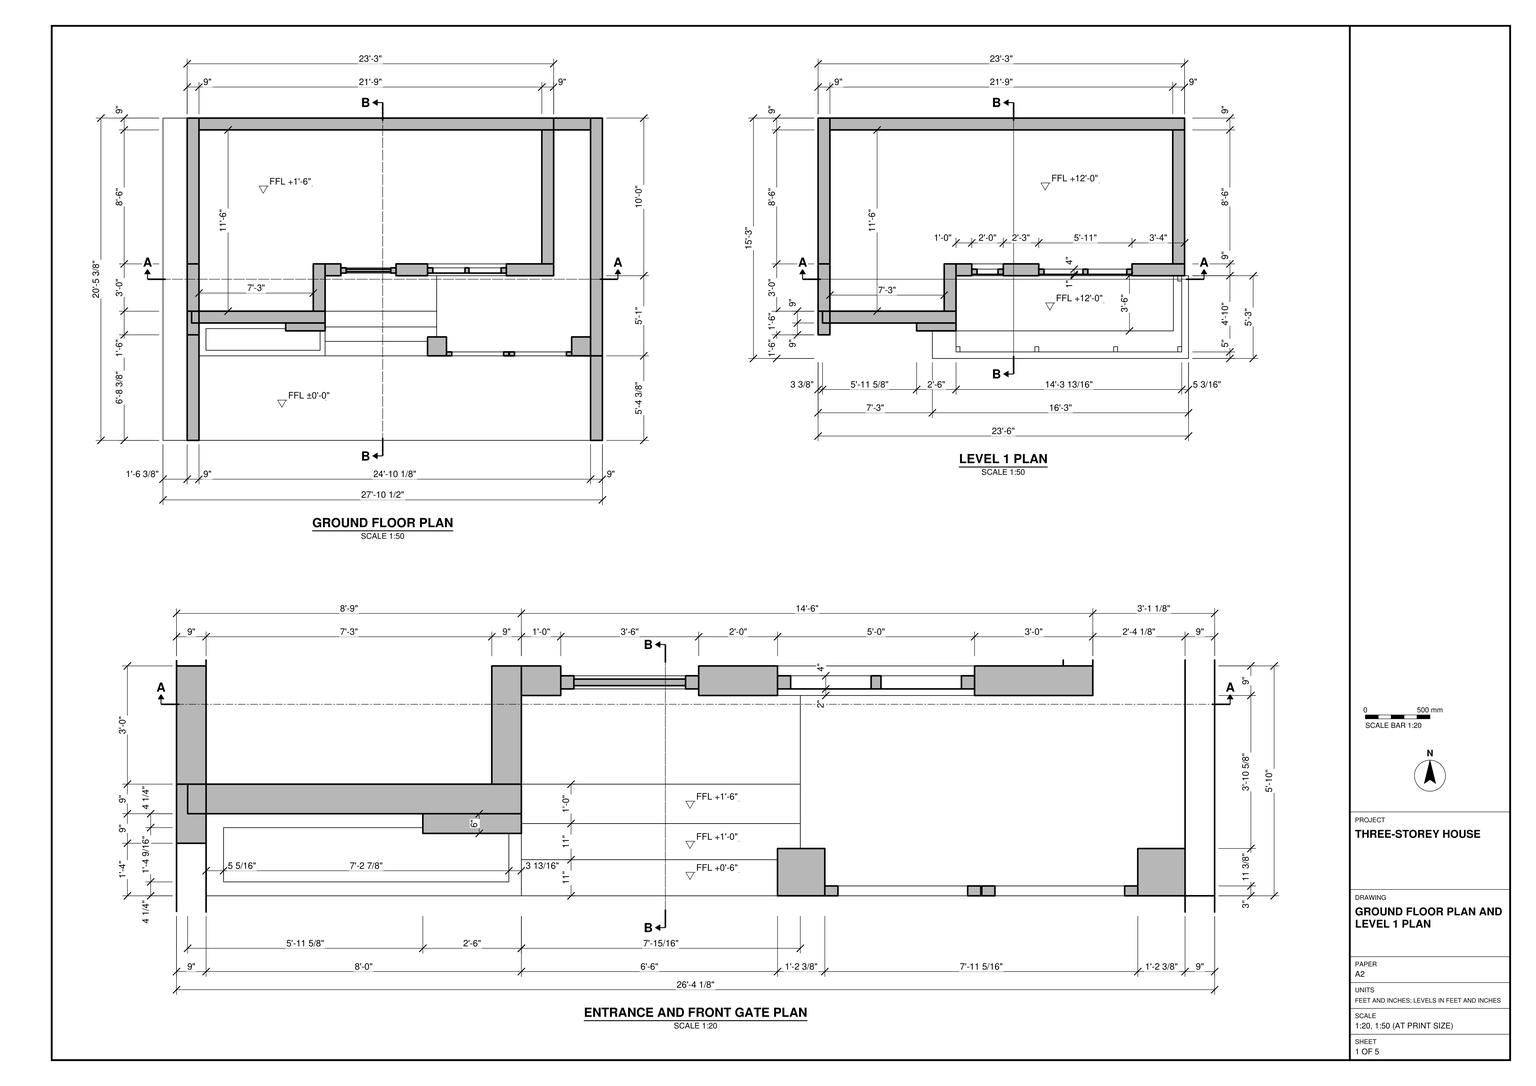
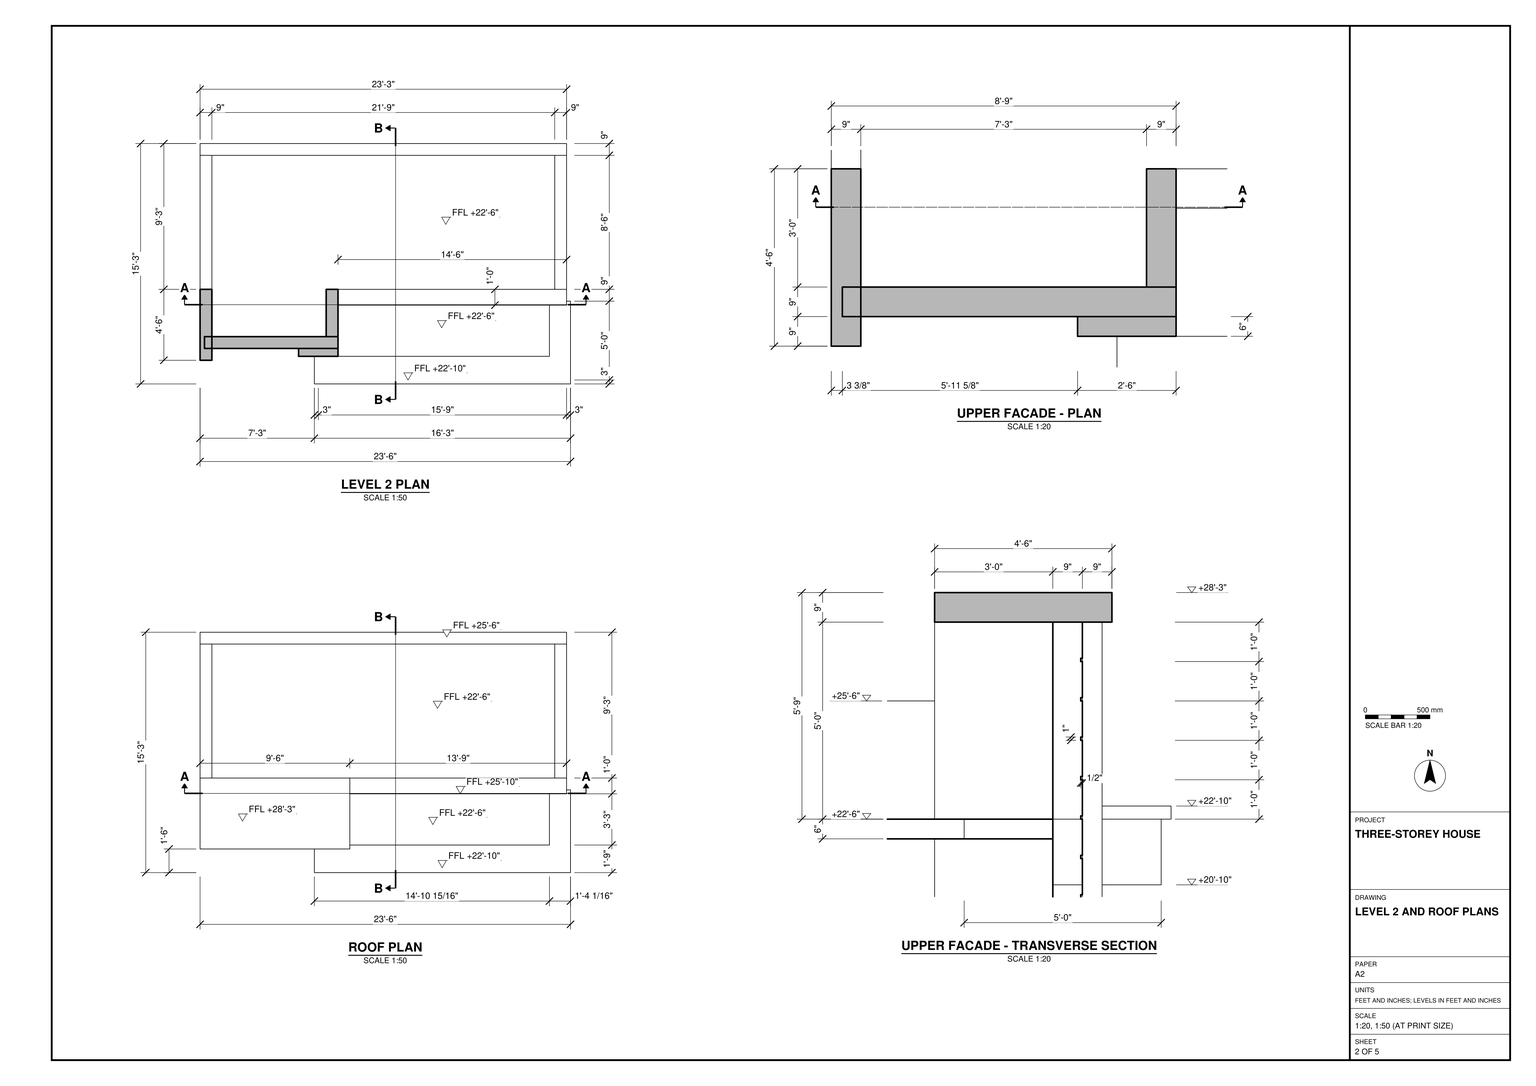
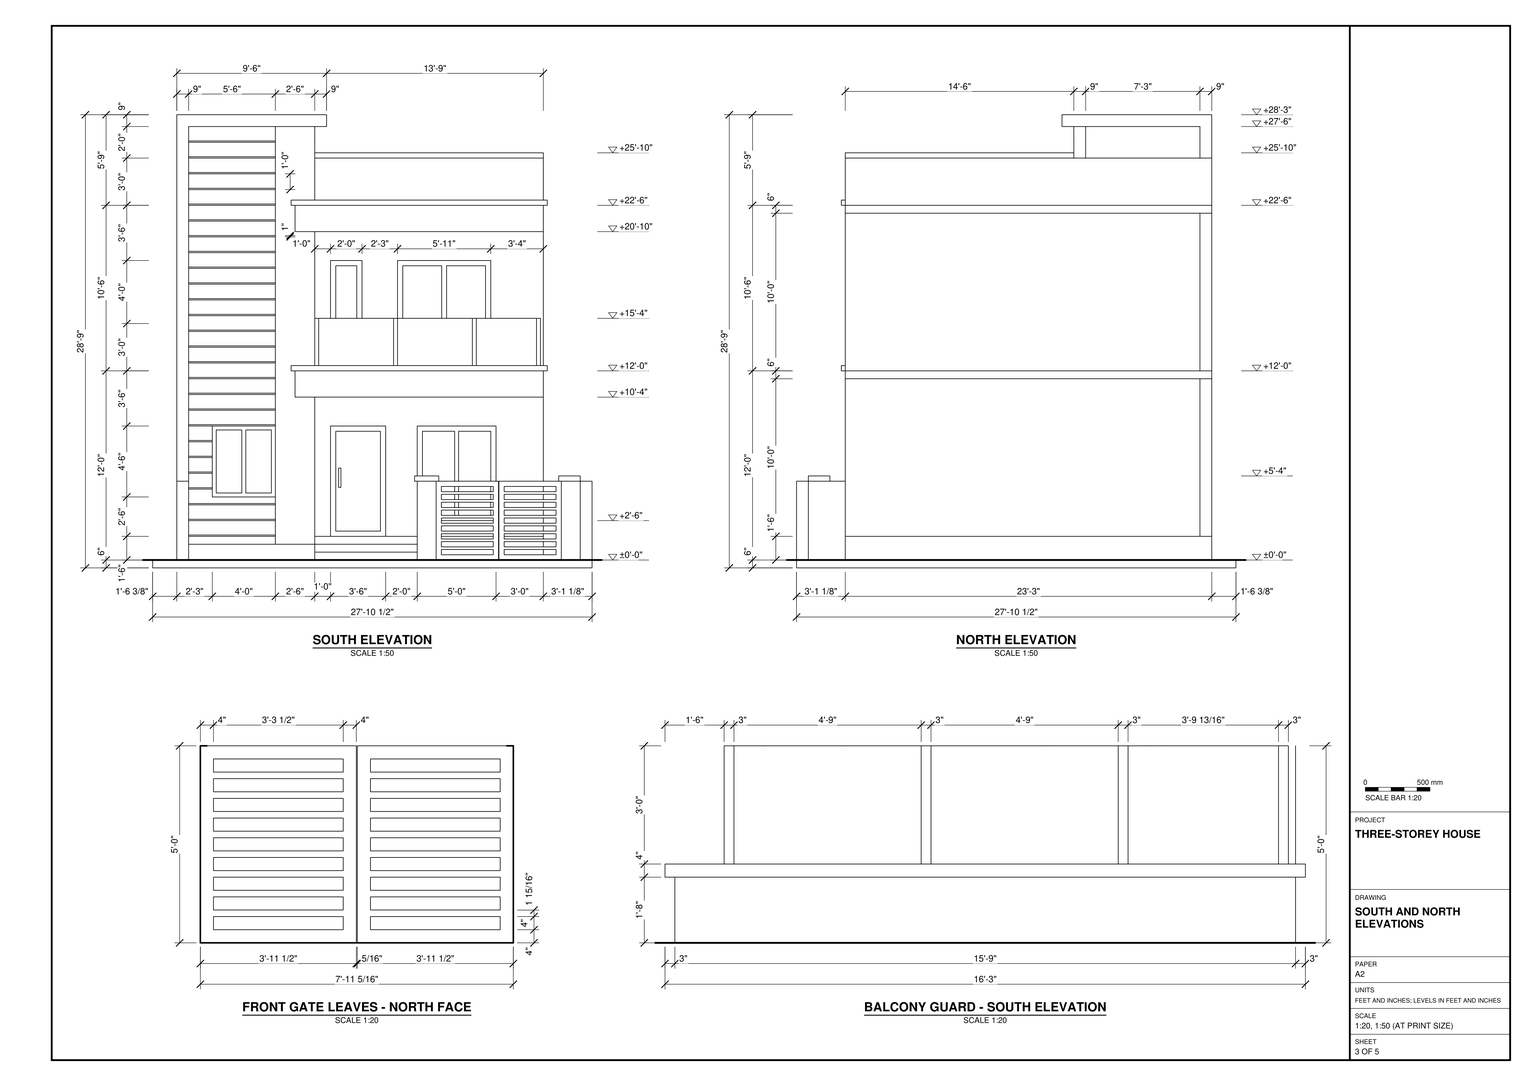
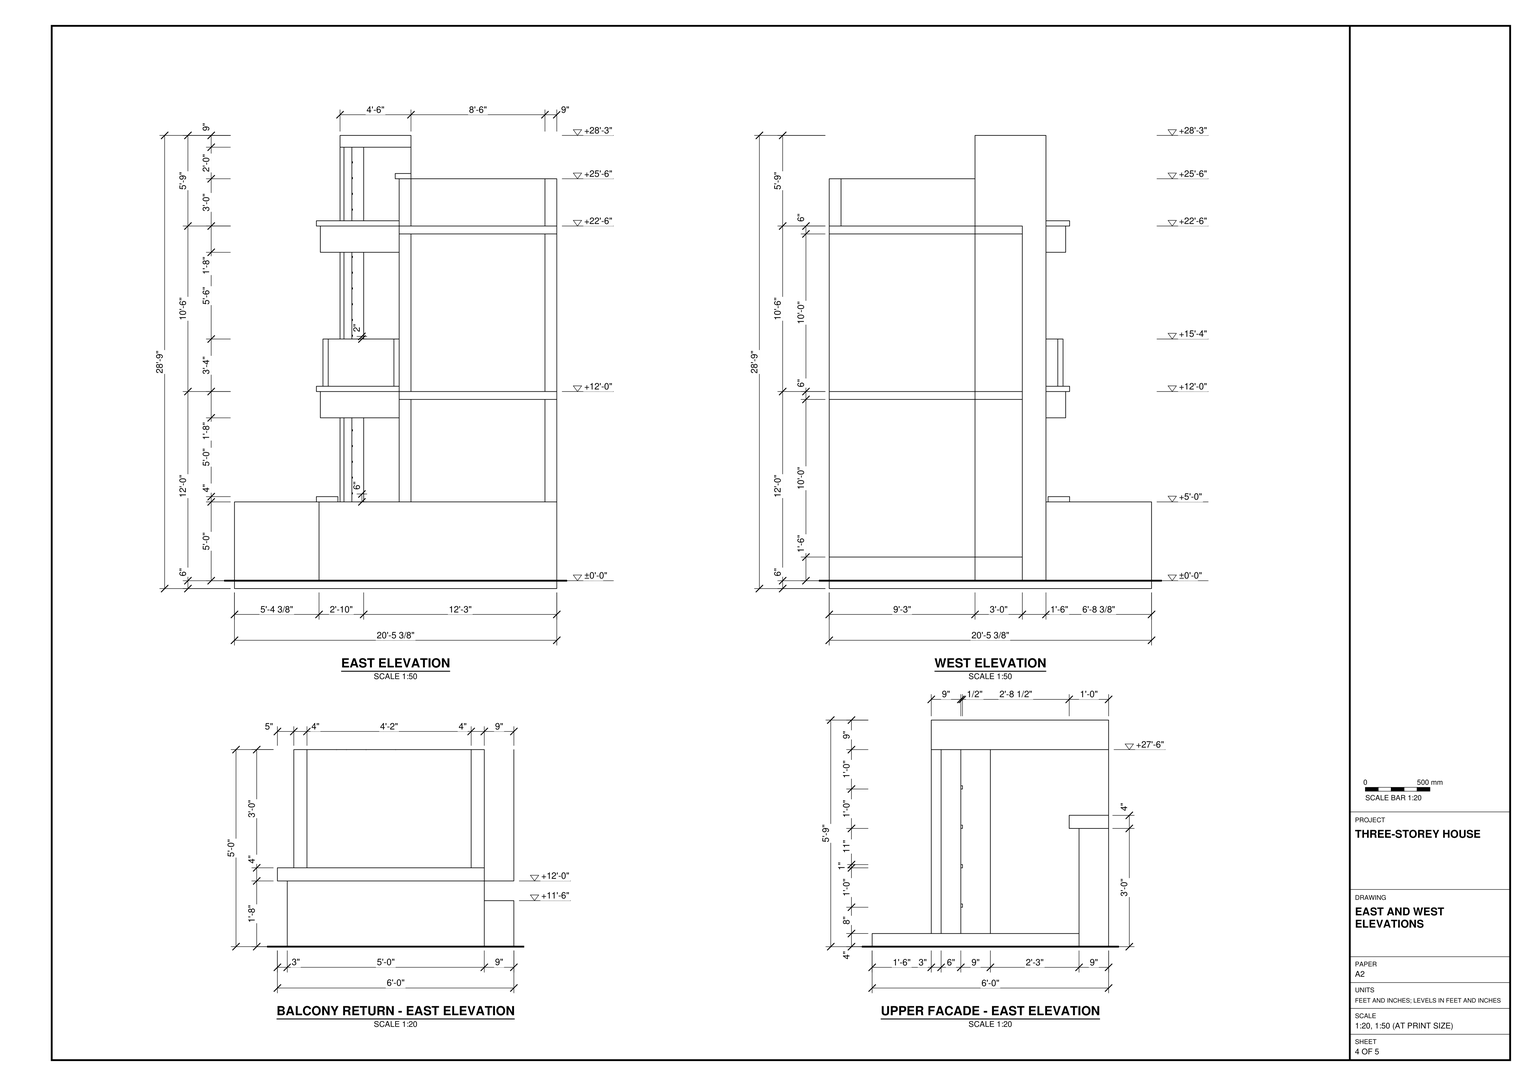
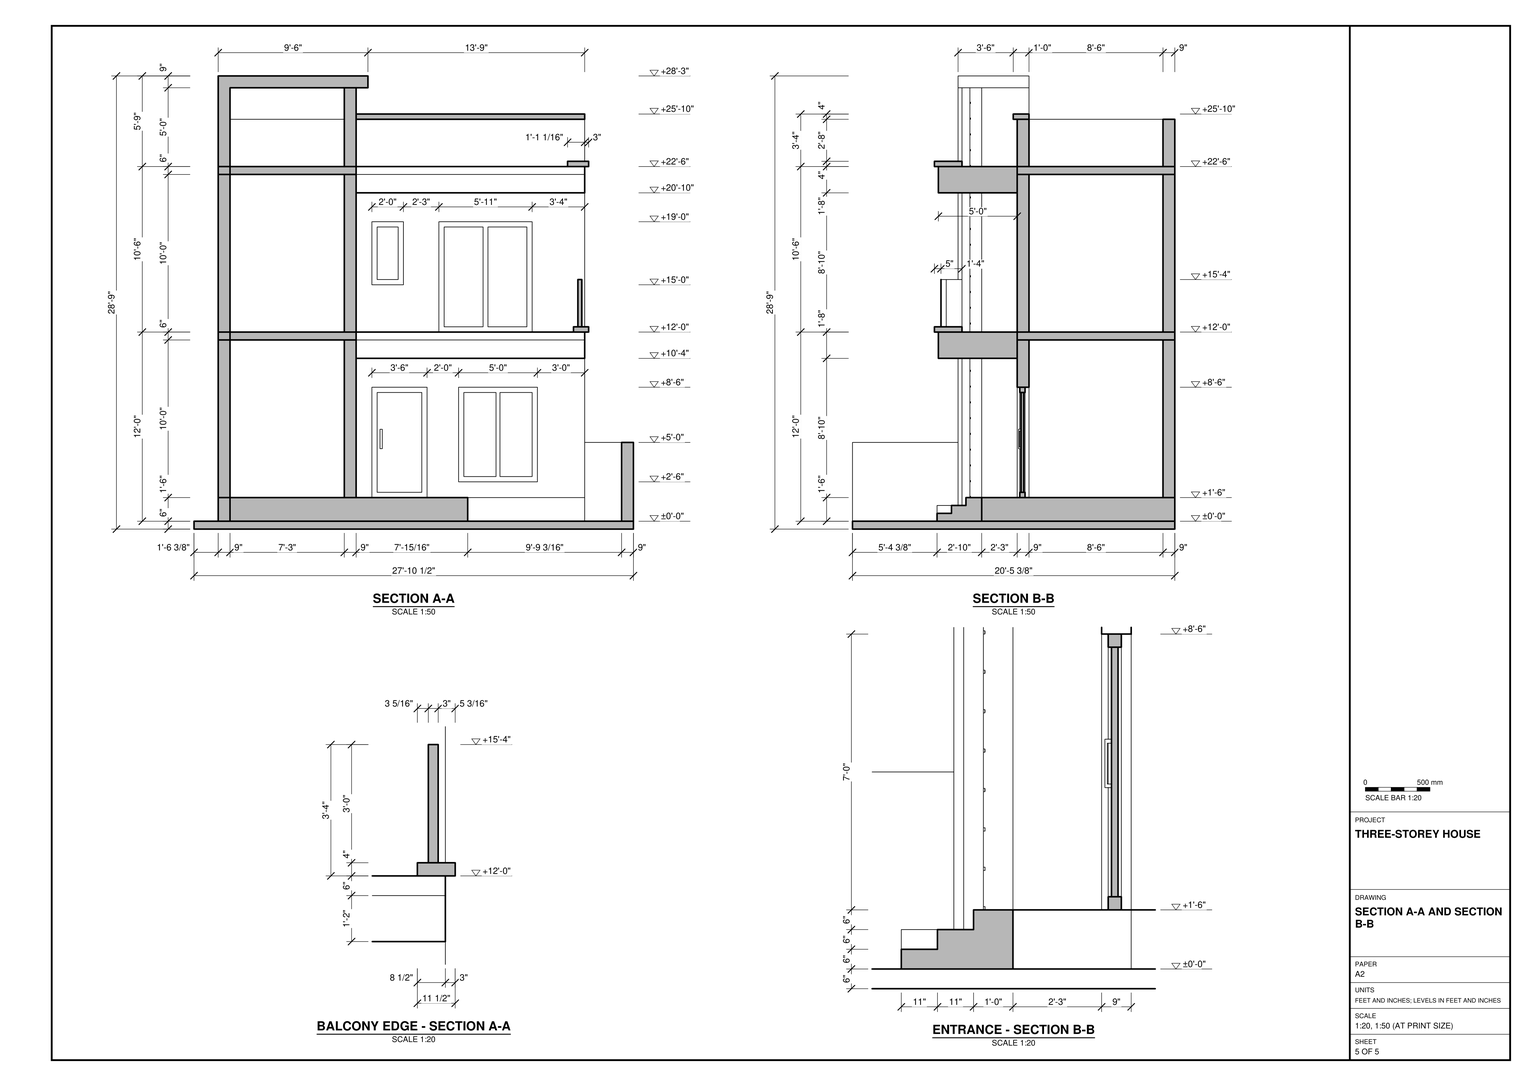
Build the house shown in task_files/diagram_01.pdf in SketchUp. Work in feet and inches. The complete model, including the base and entrance enclosure, measures 27'-10 1/2" across the south elevation, 20'-5 3/8" from front to back and 28'-9" high. Use ±0'-0" as the ground datum, with Level 1 at +12'-0" and Level 2 at +22'-6".

Follow the stepped footprint in plan, using 9" walls where indicated. Model the base, floor slabs and raised ground floor. Run the entrance steps up to the door landing at +1'-6", with the two-leaf gate between posts to the right of the steps. On the south face, distinguish the tall, horizontally banded bay on the left from the recessed door and window wall beneath the balcony. Model the openings and their frames, the projecting balcony slab and its panelled guard. Use the roof plan and transverse section to shape the flat roof, parapets and projecting cap over the tall bay.

Keep shell elements such as walls, slabs and roof separate as groups or components. Treat each furniture or joinery piece shown as a separate group or component, and use components for repeated parts. Decor and loose items may be any suitable library components. Save one SketchUp model as output_files/three_storey_house_with_a_balcony_and_gated_entrance.skp.

# SketchUp Ruby script. Lengths in inches.
U = 1.inch
M = Sketchup.active_model
def pt(a) = Geom::Point3d.new(a.map { |v| v * U })
def face(e, loops, mat)
  f = e.add_face(loops[0].map { |a| pt(a) })
  loops[1..].each { |l| e.add_face(l.map { |a| pt(a) }).erase! }
  f.material = f.back_material = mat if mat
  f
end
# faces: each face lists its corners as indices into pts; further lists are holes
def faces(e, pts, list, mat = nil) = list.each { |f| face(e, (f[0].is_a?(Array) ? f : [f]).map { |l| l.map { |i| pts[i] } }, mat) }
# xy, xz, yz: faces in a plane at the given z, y or x. An outline is a flat list of corners, or four numbers for a rectangle; further outlines are holes
def ring(l) = l.size == 4 ? [[l[0], l[1]], [l[2], l[1]], [l[2], l[3]], [l[0], l[3]]] : l.each_slice(2).to_a
def flat(e, list, mat, &to3) = list.each { |f| face(e, (f[0].is_a?(Array) ? f : [f]).map { |l| ring(l).map { |u, v| to3.(u, v) } }, mat) }
def xy(e, z, list, mat = nil) = flat(e, list, mat) { |x, y| [x, y, z] }
def xz(e, y, list, mat = nil) = flat(e, list, mat) { |x, z| [x, y, z] }
def yz(e, x, list, mat = nil) = flat(e, list, mat) { |y, z| [x, y, z] }
def lines(e, pts, list) = list.each { |a, b| e.add_line(pt(pts[a]), pt(pts[b])) }
# prism: a flat outline (further loops are holes) pulled along v
def prism(e, loops, v, mat = nil)
  f = face(e, loops, mat); d = Geom::Vector3d.new(v.map { |x| x * U })
  f.pushpull(f.normal.samedirection?(d) ? d.length : -d.length)
end
def box(e, o, s, mat = nil) = prism(e, [[o, [o[0] + s[0], o[1], o[2]], [o[0] + s[0], o[1] + s[1], o[2]], [o[0], o[1] + s[1], o[2]]]], [0, 0, s[2]], mat)
def at(x, y, z, deg = 0) = Geom::Transformation.translation(pt([x, y, z])) * Geom::Transformation.rotation(ORIGIN, Z_AXIS, deg.degrees)
def axes(o, x, y, z) = Geom::Transformation.new([*x, 0, *y, 0, *z, 0, *pt(o).to_a, 1])
def part(name) = M.definitions.add(name)
# library, detail: a bought-in or finely detailed component or shape, given as its bounding box
def library(name, o, s) = part(name).tap { |d| box(d.entities, o, s) }
def detail(e, o, s) = box(e.add_group.entities, o, s)
def put(e, d, t, mat = nil) = e.add_instance(d, t).tap { |i| i.material = mat if mat }
def group(e, t, mat = nil) = e.add_group.tap { |g| g.transformation = t; g.material = mat if mat }.entities
root = M.entities
M.materials.add("[Color M07]").color = [58, 58, 58]
M.materials.add("[Grass Dark Green]").color = [106, 157, 55]
M.materials.add("[Stone Brushed Khaki]").color = [229, 239, 196]
M.materials.add("[Translucent Glass Blue]").color = [51, 76, 122]
M.materials["[Translucent Glass Blue]"].alpha = 0.5
M.materials.add("[Translucent Glass Gray]").color = [71, 71, 71]
M.materials["[Translucent Glass Gray]"].alpha = 0.5
M.materials.add("[Translucent Glass Gray]1").color = [0, 0, 0]
M.materials["[Translucent Glass Gray]1"].alpha = 0.5
M.materials.add("[Wood Cherry Original]").color = [112, 63, 31]
M.materials.add("[Wood Veneer 01]").color = [76, 44, 23]
c1 = part("Group\#40")
box(c1.entities,[0,0,0],[3,4,36])
g1 = group(root,at(0,139,0))
box(g1,[0,-139,0],[334.5,245.37,6])
g2 = group(root,at(57.4,5.37,6))
prism(g2,[[[240,240,0],[240,120,0],[150.9375,120,0],[150.9375,93,0],[66,93,0],[-39,93,0],[-39,240,0]]],[0,0,18])
g3 = group(root,at(57.4,125.37,24))
prism(g3,[[[78,9,0],[66,9,0],[66,9,120],[240,9,120],[240,9,0],[120,9,0],[120,9,84],[78,9,84]],[[204,9,12],[204,9,84],[144,9,84],[144,9,12]]],[0,-9,0])
g4 = group(root,at(201.4,127.37,36),"[Wood Veneer 01]")
prism(g4,[[[0,0,72],[0,0,0],[60,0,0],[60,0,72]],[[28.5,0,68],[28.5,0,4],[4,0,4],[4,0,68]],[[31.5,0,68],[56,0,68],[56,0,4],[31.5,0,4]]],[0,4,0])
g5 = group(root,at(232.9,127.37,40),"[Translucent Glass Gray]")
xz(g5,0,[[0,0,24.5,64]])
g6 = group(root,at(205.4,127.37,40),"[Translucent Glass Gray]1")
xz(g6,0,[[0,0,24.5,64]])
g7 = group(root,at(135.4,127.37,24),"[Wood Veneer 01]")
prism(g7,[[[42,4,0],[0,4,0],[0,4,84],[42,4,84]],[[38,4,4],[38,4,80],[4,4,80],[4,4,4]]],[0,-4,0])
g8 = group(root,at(139.4,128.37,28),"[Wood Veneer 01]")
box(g8,[0,0,0],[34,2,76])
g9 = group(root,at(46.27,89.37,6),"[Wood Veneer 01]")
xy(g9,0,[[-24.5,0,77.125,9]])
xy(g9,6,[[-24.5,0,77.125,0.5]])
xy(g9,7,[[-24.5,0,77.125,0.5]])
xy(g9,18,[[-24.5,0,77.125,0.5]])
xy(g9,19,[[-24.5,0,77.125,0.5]])
xy(g9,30,[[-24.5,0,77.125,0.5]])
xy(g9,31,[[-24.5,0,77.125,0.5]])
xy(g9,42,[[-24.5,0,77.125,0.5]])
xy(g9,43,[[-24.5,0,77.125,0.5]])
xy(g9,48,[[-0.875,0,47.125,9]])
xy(g9,54,[[-24.5,0,-0.875,0.5],[47.125,0,77.125,0.4375]])
xy(g9,55,[[-24.5,0,-0.875,0.5],[47.125,0,77.125,0.4375]])
xy(g9,66,[[-24.5,0,-0.875,0.5],[47.125,0,77.125,0.4375]])
xy(g9,67,[[-24.5,0,-0.875,0.5],[47.125,0,77.125,0.4375]])
xy(g9,78,[[-24.5,0,-0.875,0.5],[47.125,0,77.125,0.4375]])
xy(g9,79,[[-24.5,0,-0.875,0.5],[47.125,0,77.125,0.4375]])
xy(g9,90,[[-24.5,0,-0.875,0.5],[47.125,0,77.125,0.4375]])
xy(g9,91,[[-24.5,0,-0.875,0.5],[47.125,0,77.125,0.4375]])
xy(g9,102,[[-24.5,0,-1.16,0.5],[-1.16,0,-0.875,0.5],[47.33,0,77.125,0.4375],[-0.875,0.5,47.125,9]])
xy(g9,103,[[-24.5,0,-1.16,0.5],[-1.16,0,47.125,0.5],[47.33,0,77.125,0.4375]])
xy(g9,114,[[-24.5,0,77.125,0.5]])
xy(g9,115,[[-24.5,0,77.125,0.5]])
xy(g9,126,[[-24.5,0,77.125,0.5]])
xy(g9,127,[[-24.5,0,77.125,0.5]])
xy(g9,138,[[-24.5,0,77.125,0.5]])
xy(g9,139,[[-24.5,0,77.125,0.5]])
xy(g9,150,[[-24.5,0,77.125,0.5]])
xy(g9,151,[[-24.5,0,77.125,0.5]])
xy(g9,162,[[-24.5,0,77.125,0.5]])
xy(g9,163,[[-24.5,0,77.125,0.5]])
xy(g9,174,[[-24.5,0,77.125,0.5]])
xy(g9,175,[[-24.5,0,77.125,0.5]])
xy(g9,186,[[-24.5,0,77.125,0.5]])
xy(g9,187,[[-24.5,0,77.125,0.5]])
xy(g9,198,[[-24.5,0,77.125,0.5]])
xy(g9,199,[[-24.5,0,77.125,0.5]])
xy(g9,210,[[-24.5,0,77.125,0.5]])
xy(g9,211,[[-24.5,0,77.125,0.5]])
xy(g9,222,[[-24.5,0,77.125,0.5]])
xy(g9,223,[[-24.5,0,77.125,0.5]])
xy(g9,234,[[-24.5,0,77.125,0.5]])
xy(g9,235,[[-24.5,0,77.125,0.5]])
xy(g9,246,[[-24.5,0,77.125,0.5]])
xy(g9,247,[[-24.5,0,77.125,0.5]])
xy(g9,258,[[-24.5,0,77.125,0.5]])
xy(g9,259,[[-24.5,0,77.125,0.5]])
xy(g9,270,[[-24.5,0,77.125,0.5]])
xy(g9,271,[[-24.5,0,77.125,0.5]])
xy(g9,282,[[-24.5,0,77.125,0.5]])
xy(g9,283,[[-24.5,0,77.125,0.5]])
xy(g9,294,[[-24.5,0,77.125,0.5]])
xy(g9,295,[[-24.5,0,77.125,0.5]])
xy(g9,306,[[-24.5,0,77.125,0.5]])
xy(g9,307,[[-24.5,0,77.125,0.5]])
xy(g9,318,[[-24.5,0,77.125,0.5]])
xy(g9,319,[[-24.5,0,77.125,0.5]])
xy(g9,330,[[-24.5,0,77.125,9]])
xz(g9,0,[[-24.5,0,77.125,6],[-24.5,7,77.125,18],[-24.5,19,77.125,30],[-24.5,31,77.125,42],[-24.5,43,77.125,43,77.125,54,47.125,54,47.125,48,-0.875,48,-0.875,54,-24.5,54],
  [-24.5,55,-0.875,66],[47.125,55,77.125,66],[-24.5,67,-0.875,78],[47.125,67,77.125,78],[-24.5,79,-0.875,90],
  [47.125,79,77.125,90],[-24.5,91,-0.875,102],[47.125,91,77.125,91,77.125,102,47.33,102,47.33,103,77.125,103,77.125,114,-24.5,114,-24.5,103,47.125,103],[-24.5,115,77.125,126],[-24.5,127,77.125,138],
  [-24.5,139,77.125,150],[-24.5,151,77.125,162],[-24.5,163,77.125,174],[-24.5,175,77.125,186],[-24.5,187,77.125,198],
  [-24.5,199,77.125,210],[-24.5,211,77.125,222],[-24.5,223,77.125,234],[-24.5,235,77.125,246],[-24.5,247,77.125,258],
  [-24.5,259,77.125,270],[-24.5,271,77.125,282],[-24.5,283,77.125,294],[-24.5,295,77.125,306],[-24.5,307,77.125,318],
  [-24.5,319,77.125,330]])
xz(g9,0.4375,[[47.125,54,77.125,55],[47.125,66,77.125,67],[47.125,78,77.125,79],[47.125,90,77.125,91],[47.33,102,77.125,103]])
xz(g9,0.5,[[-24.5,6,77.125,7],[-24.5,18,77.125,19],[-24.5,30,77.125,31],[-24.5,42,77.125,43],[-24.5,54,-0.875,55],
  [-24.5,66,-0.875,67],[-24.5,78,-0.875,79],[-24.5,90,-0.875,91],[-24.5,102,47.125,103],[-24.5,114,77.125,115],
  [-24.5,126,77.125,127],[-24.5,138,77.125,139],[-24.5,150,77.125,151],[-24.5,162,77.125,163],[-24.5,174,77.125,175],
  [-24.5,186,77.125,187],[-24.5,198,77.125,199],[-24.5,210,77.125,211],[-24.5,222,77.125,223],[-24.5,234,77.125,235],
  [-24.5,246,77.125,247],[-24.5,258,77.125,259],[-24.5,270,77.125,271],[-24.5,282,77.125,283],[-24.5,294,77.125,295],
  [-24.5,306,77.125,307],[-24.5,318,77.125,319]])
xz(g9,9,[[[-24.5,0,77.125,330],[-0.875,48,47.125,102]]])
yz(g9,-24.5,[[0,0,0,6,0.5,6,0.5,7,0,7,0,18,0.5,18,0.5,19,0,19,0,30,0.5,30,0.5,31,0,31,0,42,0.5,42,0.5,43,0,43,0,54,0.5,54,0.5,55,0,55,0,66,0.5,66,0.5,67,0,67,0,78,0.5,78,0.5,79,0,79,0,90,0.5,90,0.5,91,0,91,0,102,0.5,102,0.5,103,0,103,0,114,0.5,114,0.5,115,0,115,0,126,0.5,126,0.5,127,0,127,0,138,0.5,138,0.5,139,0,139,0,150,0.5,150,0.5,151,0,151,0,162,0.5,162,0.5,163,0,163,0,174,0.5,174,0.5,175,0,175,0,186,0.5,186,0.5,187,0,187,0,198,0.5,198,0.5,199,0,199,0,210,0.5,210,0.5,211,0,211,0,222,0.5,222,0.5,223,0,223,0,234,0.5,234,0.5,235,0,235,0,246,0.5,246,0.5,247,0,247,0,258,0.5,258,0.5,259,0,259,0,270,0.5,270,0.5,271,0,271,0,282,0.5,282,0.5,283,0,283,0,294,0.5,294,0.5,295,0,295,0,306,0.5,306,0.5,307,0,307,0,318,0.5,318,0.5,319,0,319,0,330,9,330,9,0]])
yz(g9,-0.875,[[0,48,9,48,9,102,0,102,0,91,0.5,91,0.5,90,0,90,0,79,0.5,79,0.5,78,0,78,0,67,0.5,67,0.5,66,0,66,0,55,0.5,55,0.5,54,0,54]])
yz(g9,47.125,[[0,48,0,54,0.4375,54,0.4375,55,0,55,0,66,0.4375,66,0.4375,67,0,67,0,78,0.4375,78,0.4375,79,0,79,0,90,0.4375,90,0.4375,91,0,91,0,102,9,102,9,48],[0,102,0.5,103]])
yz(g9,47.33,[[0,102,0.4375,103]])
yz(g9,77.125,[[0,0,9,0,9,330,0,330,0,319,0.5,319,0.5,318,0,318,0,307,0.5,307,0.5,306,0,306,0,295,0.5,295,0.5,294,0,294,0,283,0.5,283,0.5,282,0,282,0,271,0.5,271,0.5,270,0,270,0,259,0.5,259,0.5,258,0,258,0,247,0.5,247,0.5,246,0,246,0,235,0.5,235,0.5,234,0,234,0,223,0.5,223,0.5,222,0,222,0,211,0.5,211,0.5,210,0,210,0,199,0.5,199,0.5,198,0,198,0,187,0.5,187,0.5,186,0,186,0,175,0.5,175,0.5,174,0,174,0,163,0.5,163,0.5,162,0,162,0,151,0.5,151,0.5,150,0,150,0,139,0.5,139,0.5,138,0,138,0,127,0.5,127,0.5,126,0,126,0,115,0.5,115,0.5,114,0,114,0,103,0.4375,103,0.4375,102,0,102,0,91,0.4375,91,0.4375,90,0,90,0,79,0.4375,79,0.4375,78,0,78,0,67,0.4375,67,0.4375,66,0,66,0,55,0.4375,55,0.4375,54,0,54,0,43,0.5,43,0.5,42,0,42,0,31,0.5,31,0.5,30,0,30,0,19,0.5,19,0.5,18,0,18,0,7,0.5,7,0.5,6,0,6]])
g10 = group(root,at(114.4,98.37,24),"[Wood Veneer 01]")
box(g10,[0,0,0],[9,36,120])
g11 = group(root,at(45.4,93.87,54),"[Wood Cherry Original]")
prism(g11,[[[48,4,54],[48,4,0],[0,4,0],[0,4,54]],[[22.5,4,3],[22.5,4,51],[3,4,51],[3,4,3]],[[45,4,51],[25.5,4,51],[25.5,4,3],[45,4,3]]],[0,-4,0])
g12 = group(root,at(70.9,93.87,57),"[Translucent Glass Gray]1")
xz(g12,0,[[0,0,19.5,48]])
g13 = group(root,at(48.4,93.87,57),"[Translucent Glass Gray]1")
xz(g13,0,[[0,0,19.5,48]])
g14 = group(root,at(18.4,98.37,24))
box(g14,[0,0,0],[9,147,120])
g15 = group(root,at(27.4,236.37,24))
box(g15,[0,0,0],[270,9,120])
g16 = group(root,at(288.4,134.37,24))
box(g16,[0,0,0],[9,102,120])
g17 = group(root,at(18.4,98.37,144))
prism(g17,[[[279,147,0],[279,27,0],[105,27,0],[105,0,0],[0,0,0],[0,147,0]]],[0,0,6])
g18 = group(root,at(123.4,89.37,130))
xy(g18,0,[[-15,-24,-15,-6,0,-6,0,36,174,36,174,-24]],"[Wood Veneer 01]")
xy(g18,20,[[-15,-24,174,-24,174,36,0,36,0,-6,-15,-6]])
xz(g18,-24,[[-15,0,174,20]])
xz(g18,-6,[[-15,0,0,20]])
xz(g18,36,[[0,0,174,20]])
yz(g18,-15,[[-24,0,-6,20]])
yz(g18,0,[[-6,0,36,20]])
yz(g18,174,[[-24,0,36,20]])
g19 = group(root,at(123.4,125.37,150))
prism(g19,[[[63,9,0],[0,9,0],[0,9,120],[174,9,120],[174,9,0],[134,9,0],[134,9,84],[63,9,84]],[[36,9,36],[36,9,84],[12,9,84],[12,9,36]]],[0,-9,0])
g20 = group(root,at(186.4,126.37,150),"[Wood Veneer 01]")
prism(g20,[[[71,4,0],[0,4,0],[0,4,84],[71,4,84]],[[33.65,4,4],[33.65,4,80],[4,4,80],[4,4,4]],[[67,4,80],[37.35,4,80],[37.35,4,4],[67,4,4]]],[0,-4,0])
g21 = group(root,at(223.75,126.37,154),"[Translucent Glass Blue]")
xz(g21,0,[[0,0,29.65,76]])
g22 = group(root,at(190.4,126.37,154),"[Translucent Glass Blue]")
xz(g22,0,[[0,0,29.65,76]])
g23 = group(root,at(135.4,126.37,186),"[Wood Veneer 01]")
prism(g23,[[[0,0,48],[0,0,0],[24,0,0],[24,0,48]],[[20,0,44],[20,0,4],[4,0,4],[4,0,44]]],[0,4,0])
g24 = group(root,at(139.4,126.37,190),"[Translucent Glass Blue]")
xz(g24,0,[[0,0,16,40]])
g25 = group(root,at(114.4,98.37,150),"[Wood Veneer 01]")
box(g25,[0,0,0],[9,36,120])
g26 = group(root,at(18.4,98.37,150))
box(g26,[0,0,0],[9,147,120])
g27 = group(root,at(27.4,236.37,150))
box(g27,[0,0,0],[270,9,120])
g28 = group(root,at(288.4,134.37,150))
box(g28,[0,0,0],[9,102,120])
g29 = group(root,at(18.4,98.37,270))
prism(g29,[[[0,147,0],[279,147,0],[279,27,0],[105,27,0],[105,0,0],[0,0,0]]],[0,0,6])
g30 = group(root,at(123.4,89.37,256))
xy(g30,0,[[-15,-24,-15,-6,0,-6,0,36,174,36,174,-24]],"[Wood Veneer 01]")
xy(g30,20,[[-15,-24,174,-24,174,36,0,36,0,-6,-15,-6]])
xz(g30,-24,[[-15,0,174,20]])
xz(g30,-6,[[-15,0,0,20]])
xz(g30,36,[[0,0,174,20]])
yz(g30,-15,[[-24,0,-6,20]])
yz(g30,0,[[-6,0,36,20]])
yz(g30,174,[[-24,0,36,20]])
g31 = group(root,at(123.4,125.37,276))
box(g31,[0,0,0],[174,9,36])
g32 = group(root,at(288.4,134.37,276))
box(g32,[0,0,0],[9,102,36])
g33 = group(root,at(18.4,236.37,276))
box(g33,[0,0,0],[279,9,36])
g34 = group(root,at(114.4,98.37,276),"[Wood Veneer 01]")
box(g34,[0,0,0],[9,36,60])
g35 = group(root,at(93.4,83.37,6),"[Wood Veneer 01]")
box(g35,[0,0,0],[30,6,330])
g36 = group(root,at(18.4,80.37,6))
prism(g36,[[[9,0,0],[9,0,330],[114,0,330],[114,0,339],[0,0,339],[0,0,0]]],[0,54,0])
g37 = group(root,at(108.4,65.37,276))
prism(g37,[[[-3,-3,0],[-3,18,0],[175.96,18,0],[175.96,60,0],[192,60,0],[192,-3,0]]],[0,0,4])
g38 = group(root,at(123.4,122.37,312))
box(g38,[0,0,0],[174,12,4])
g39 = group(root,at(108.4,65.37,150))
prism(g39,[[[192,60,0],[192,-3,0],[-3,-3,0],[-3,18,0],[180.47,18,0],[180.47,60,0]]],[0,0,4])
put(root,c1,at(123.4,67.37,154),"[Color M07]")
put(root,c1,at(183.4,67.37,154),"[Color M07]")
put(root,c1,at(243.4,67.37,154),"[Color M07]")
put(root,c1,at(292.21,67.37,154),"[Color M07]")
put(root,c1,at(292.21,121.37,154),"[Color M07]")
g40 = group(root,at(123.4,71.37,154),"[Translucent Glass Gray]1")
yz(g40,0,[[0,0,12,36]])
g41 = group(root,at(295.21,71.37,154),"[Translucent Glass Gray]1")
yz(g41,0,[[0,0,50,36]])
g42 = group(root,at(246.4,67.37,154),"[Translucent Glass Gray]1")
xz(g42,0,[[0,0,45.8125,36]])
g43 = group(root,at(186.4,67.37,154),"[Translucent Glass Gray]1")
xz(g43,0,[[0,0,57,36]])
g44 = group(root,at(126.4,67.37,154),"[Translucent Glass Gray]1")
xz(g44,0,[[0,0,57,36]])
g45 = group(root,at(123.4,64.37,6),"[Stone Brushed Khaki]")
xy(g45,0,[[0,0,0,34,84.9375,34,84.9375,14.4,78,14.4,78,0]])
xy(g45,6,[[0,0,78,11]])
xy(g45,12,[[0,11,78,11,78,14.4,84.9375,14.4,84.9375,22,0,22]])
xy(g45,18,[[0,22,84.9375,34]])
xz(g45,0,[[0,0,78,6]])
xz(g45,11,[[0,6,78,12]])
xz(g45,14.4,[[78,0,84.9375,12]])
xz(g45,22,[[0,12,84.9375,18]])
xz(g45,34,[[0,0,84.9375,18]])
yz(g45,0,[[0,0,0,6,11,6,11,12,22,12,22,18,34,18,34,0]])
yz(g45,78,[[0,0,14.4,0,14.4,12,11,12,11,6,0,6]])
yz(g45,84.9375,[[14.4,0,34,0,34,18,22,18,22,12,14.4,12]])
g46 = group(root,at(201.4,64.37,6))
box(g46,[0,0,0],[14.4,14.4,60])
g47 = group(root,at(311.1,64.37,6))
box(g47,[0,0,0],[14.4,14.4,60])
g48 = group(root,at(215.8,64.37,6),"[Color M07]")
prism(g48,[[[47.8,0,0],[95.3,0,0],[95.3,0,60],[47.8,0,60]],[[91.3,0,52],[51.8,0,52],[51.8,0,56],[91.3,0,56]],[[91.3,0,40],[51.8,0,40],[51.8,0,44],[91.3,0,44]],[[51.8,0,46],[51.8,0,50],[91.3,0,50],[91.3,0,46]],[[91.3,0,28],[51.8,0,28],[51.8,0,32],[91.3,0,32]],[[51.8,0,34],[51.8,0,38],[91.3,0,38],[91.3,0,34]],[[91.3,0,16],[51.8,0,16],[51.8,0,20],[91.3,0,20]],[[51.8,0,22],[51.8,0,26],[91.3,0,26],[91.3,0,22]],[[51.8,0,8],[91.3,0,8],[91.3,0,4],[51.8,0,4]],[[51.8,0,10],[51.8,0,14],[91.3,0,14],[91.3,0,10]]],[0,3,0])
prism(g48,[[[0,3,60],[47.5,3,60],[47.5,3,0],[0,3,0]],[[4,3,52],[43.5,3,52],[43.5,3,56],[4,3,56]],[[4,3,40],[43.5,3,40],[43.5,3,44],[4,3,44]],[[4,3,50],[4,3,46],[43.5,3,46],[43.5,3,50]],[[4,3,28],[43.5,3,28],[43.5,3,32],[4,3,32]],[[4,3,38],[4,3,34],[43.5,3,34],[43.5,3,38]],[[4,3,22],[43.5,3,22],[43.5,3,26],[4,3,26]],[[4,3,10],[43.5,3,10],[43.5,3,14],[4,3,14]],[[4,3,20],[4,3,16],[43.5,3,16],[43.5,3,20]],[[43.5,3,4],[43.5,3,8],[4,3,8],[4,3,4]]],[0,-3,0])
g49 = group(root,at(325.5,64.37,6))
box(g49,[0,0,0],[9,181,60])
g50 = group(root,at(297.4,236.37,6))
box(g50,[0,0,0],[28.1,9,60])
g51 = group(root,at(18.4,64.37,6))
xy(g51,0,[[9,0,105,25]])
xy(g51,10.6875,[[14.31,4.23,101.19,20.77]],"[Grass Dark Green]")
xy(g51,12,[[[9,0,105,25],[14.31,4.23,101.19,20.77]]])
xz(g51,0,[[9,0,105,12]])
xz(g51,4.23,[[14.31,10.6875,101.19,12]])
xz(g51,20.77,[[14.31,10.6875,101.19,12]])
xz(g51,25,[[9,0,105,12]])
yz(g51,9,[[0,0,25,12]])
yz(g51,14.31,[[4.23,10.6875,20.77,12]])
yz(g51,101.19,[[4.23,10.6875,20.77,12]])
yz(g51,105,[[0,0,25,12]])
g52 = group(root,at(18.4,0,6))
box(g52,[0,0,0],[9,80.37,60])
g53 = group(root,at(325.5,0,6))
box(g53,[0,0,0],[9,64.37,60])
g54 = group(root,at(199.4,62.37,66))
box(g54,[0,0,0],[18.4,16.4,4])
g55 = group(root,at(309.1,62.37,66))
box(g55,[0,0,0],[16.4,16.4,4])
g56 = group(root,at(141.57,126.37,61.23))
prism(g56,[[[0,0.73,1.1],[0,2,1.1],[0,2,0],[0,0,0],[0,0,14.75],[0,2,14.75],[0,2,13.52],[0,0.73,13.52]]],[1.75,0,0])
g57 = group(root,at(18.4,134.37,276))
box(g57,[0,0,0],[9,102,36])
